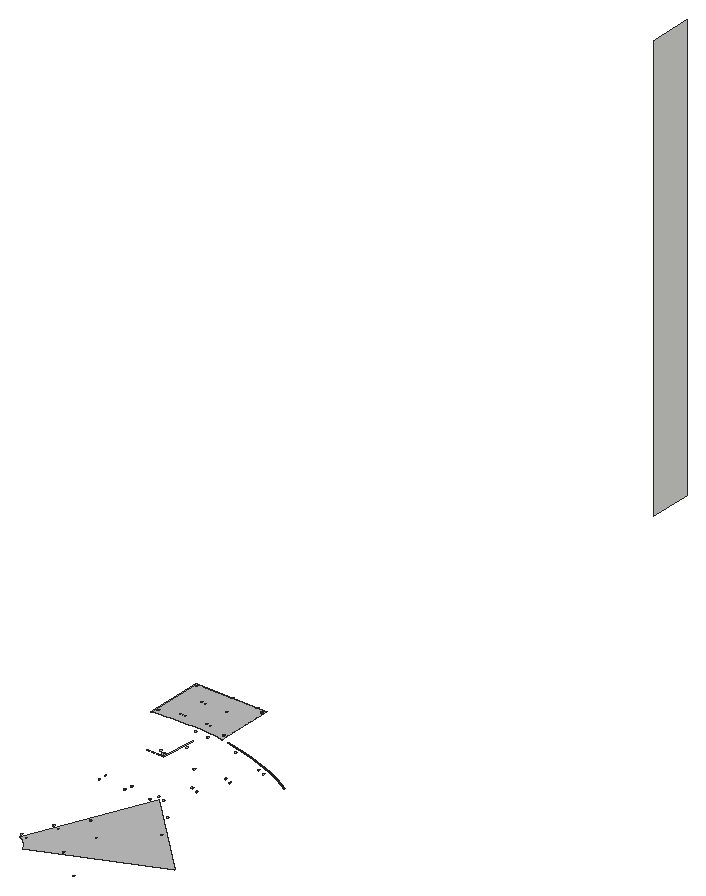
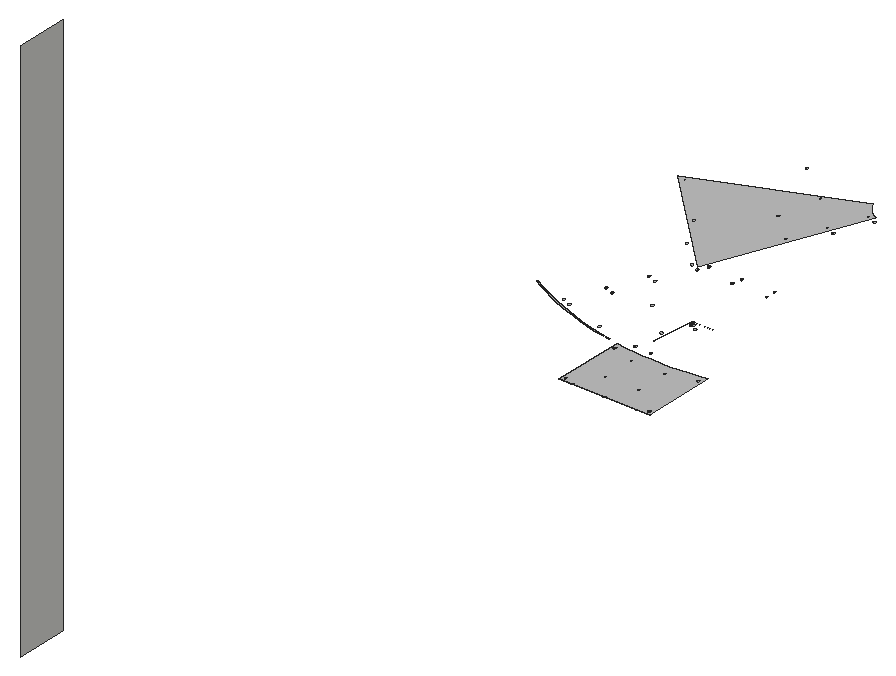
# SketchUp Ruby script. Lengths in inches.
U = 1.inch
M = Sketchup.active_model
def pt(a) = Geom::Point3d.new(a.map { |v| v * U })
def face(e, loops, mat)
  f = e.add_face(loops[0].map { |a| pt(a) })
  loops[1..].each { |l| e.add_face(l.map { |a| pt(a) }).erase! }
  f.material = f.back_material = mat if mat
  f
end
# faces: each face lists its corners as indices into pts; further lists are holes
def faces(e, pts, list, mat = nil) = list.each { |f| face(e, (f[0].is_a?(Array) ? f : [f]).map { |l| l.map { |i| pts[i] } }, mat) }
# xy, xz, yz: faces in a plane at the given z, y or x. An outline is a flat list of corners, or four numbers for a rectangle; further outlines are holes
def ring(l) = l.size == 4 ? [[l[0], l[1]], [l[2], l[1]], [l[2], l[3]], [l[0], l[3]]] : l.each_slice(2).to_a
def flat(e, list, mat, &to3) = list.each { |f| face(e, (f[0].is_a?(Array) ? f : [f]).map { |l| ring(l).map { |u, v| to3.(u, v) } }, mat) }
def xy(e, z, list, mat = nil) = flat(e, list, mat) { |x, y| [x, y, z] }
def xz(e, y, list, mat = nil) = flat(e, list, mat) { |x, z| [x, y, z] }
def yz(e, x, list, mat = nil) = flat(e, list, mat) { |y, z| [x, y, z] }
def lines(e, pts, list) = list.each { |a, b| e.add_line(pt(pts[a]), pt(pts[b])) }
# prism: a flat outline (further loops are holes) pulled along v
def prism(e, loops, v, mat = nil)
  f = face(e, loops, mat); d = Geom::Vector3d.new(v.map { |x| x * U })
  f.pushpull(f.normal.samedirection?(d) ? d.length : -d.length)
end
def box(e, o, s, mat = nil) = prism(e, [[o, [o[0] + s[0], o[1], o[2]], [o[0] + s[0], o[1] + s[1], o[2]], [o[0], o[1] + s[1], o[2]]]], [0, 0, s[2]], mat)
def at(x, y, z, deg = 0) = Geom::Transformation.translation(pt([x, y, z])) * Geom::Transformation.rotation(ORIGIN, Z_AXIS, deg.degrees)
def axes(o, x, y, z) = Geom::Transformation.new([*x, 0, *y, 0, *z, 0, *pt(o).to_a, 1])
def part(name) = M.definitions.add(name)
# library, detail: a bought-in or finely detailed component or shape, given as its bounding box
def library(name, o, s) = part(name).tap { |d| box(d.entities, o, s) }
def detail(e, o, s) = box(e.add_group.entities, o, s)
def put(e, d, t, mat = nil) = e.add_instance(d, t).tap { |i| i.material = mat if mat }
def group(e, t, mat = nil) = e.add_group.tap { |g| g.transformation = t; g.material = mat if mat }.entities
root = M.entities
M.materials.add("[Metal_Steel_Textured_White]").color = [191, 191, 191]
xy(root,3.625,[[158.645,163.377,158.648,163.4,158.657,163.422,158.671,163.44,158.689,163.454,158.711,163.463,158.734,163.466,158.757,163.463,158.778,163.454,158.797,163.44,158.811,163.422,158.82,163.4,158.823,163.377,158.822,163.377,158.819,163.4,158.81,163.421,158.796,163.44,158.778,163.454,158.757,163.462,158.734,163.465,158.711,163.462,158.69,163.454,158.672,163.44,158.658,163.421,158.649,163.4,158.646,163.377],[[152.277,164.396,152.205,164.555,152.123,164.708,152.031,164.856,151.929,164.998,151.819,165.132,151.7,165.259,151.573,165.378,151.438,165.489,151.297,165.59,151.149,165.682,150.995,165.764,150.836,165.836,156.019,178.348,164.789,169.578],[151.348,165.939,151.371,165.942,151.392,165.951,151.411,165.965,151.425,165.984,151.434,166.005,151.437,166.028,151.434,166.051,151.425,166.073,151.411,166.091,151.392,166.105,151.371,166.114,151.348,166.117,151.325,166.114,151.304,166.105,151.285,166.091,151.271,166.073,151.262,166.051,151.259,166.028,151.262,166.005,151.271,165.984,151.285,165.965,151.304,165.951,151.325,165.942],[156.159,177.554,156.182,177.557,156.204,177.566,156.222,177.58,156.236,177.599,156.245,177.62,156.248,177.643,156.245,177.666,156.236,177.688,156.222,177.706,156.204,177.72,156.182,177.729,156.159,177.732,156.136,177.729,156.115,177.72,156.096,177.706,156.082,177.688,156.073,177.666,156.07,177.643,156.073,177.62,156.082,177.599,156.096,177.58,156.115,177.566,156.136,177.557],[162.103,171.611,162.126,171.614,162.147,171.623,162.165,171.637,162.18,171.655,162.189,171.677,162.192,171.7,162.189,171.723,162.18,171.744,162.165,171.763,162.147,171.777,162.126,171.786,162.103,171.789,162.08,171.786,162.058,171.777,162.04,171.763,162.026,171.744,162.017,171.723,162.014,171.7,162.017,171.677,162.026,171.655,162.04,171.637,162.058,171.623,162.08,171.614],[154.956,174.651,154.979,174.654,155.001,174.663,155.019,174.677,155.033,174.695,155.042,174.717,155.045,174.74,155.042,174.763,155.033,174.784,155.019,174.802,155.001,174.817,154.979,174.825,154.956,174.828,154.933,174.825,154.912,174.817,154.893,174.802,154.879,174.784,154.87,174.763,154.867,174.74,154.87,174.717,154.879,174.695,154.893,174.677,154.912,174.663,154.933,174.654],[160.121,173.592,160.144,173.595,160.166,173.604,160.184,173.618,160.198,173.637,160.207,173.658,160.21,173.681,160.207,173.704,160.198,173.725,160.184,173.744,160.166,173.758,160.144,173.767,160.121,173.77,160.098,173.767,160.077,173.758,160.059,173.744,160.044,173.725,160.036,173.704,160.033,173.681,160.036,173.658,160.044,173.637,160.059,173.618,160.077,173.604,160.098,173.595],[153.754,171.747,153.777,171.75,153.798,171.759,153.816,171.773,153.831,171.791,153.839,171.813,153.842,171.836,153.839,171.859,153.831,171.88,153.816,171.899,153.798,171.913,153.777,171.922,153.754,171.925,153.731,171.922,153.709,171.913,153.691,171.899,153.677,171.88,153.668,171.859,153.665,171.836,153.668,171.813,153.677,171.791,153.691,171.773,153.709,171.759,153.731,171.75],[158.14,175.573,158.163,175.576,158.185,175.585,158.203,175.599,158.217,175.618,158.226,175.639,158.229,175.662,158.226,175.685,158.217,175.707,158.203,175.725,158.185,175.739,158.163,175.748,158.14,175.751,158.117,175.748,158.096,175.739,158.077,175.725,158.063,175.707,158.054,175.685,158.051,175.662,158.054,175.639,158.063,175.618,158.077,175.599,158.096,175.585,158.117,175.576],[155.372,166.021,155.395,166.024,155.417,166.033,155.435,166.047,155.449,166.066,155.458,166.087,155.461,166.11,155.458,166.133,155.449,166.155,155.435,166.173,155.417,166.187,155.395,166.196,155.372,166.199,155.349,166.196,155.328,166.187,155.31,166.173,155.295,166.155,155.287,166.133,155.284,166.11,155.287,166.087,155.295,166.066,155.31,166.047,155.328,166.033,155.349,166.024],[164.084,169.63,164.107,169.633,164.128,169.642,164.147,169.656,164.161,169.674,164.17,169.696,164.173,169.719,164.17,169.742,164.161,169.763,164.147,169.782,164.128,169.796,164.107,169.805,164.084,169.808,164.061,169.805,164.039,169.796,164.021,169.782,164.007,169.763,163.998,169.742,163.995,169.719,163.998,169.696,164.007,169.674,164.021,169.656,164.039,169.642,164.061,169.633],[152.469,164.819,152.492,164.822,152.513,164.831,152.532,164.845,152.546,164.863,152.555,164.885,152.558,164.908,152.555,164.931,152.546,164.952,152.532,164.97,152.513,164.984,152.492,164.993,152.469,164.996,152.446,164.993,152.424,164.984,152.406,164.97,152.392,164.952,152.383,164.931,152.38,164.908,152.383,164.885,152.392,164.863,152.406,164.845,152.424,164.831,152.446,164.822],[161.18,168.427,161.203,168.43,161.224,168.439,161.243,168.453,161.257,168.471,161.266,168.493,161.269,168.516,161.266,168.539,161.257,168.56,161.243,168.579,161.224,168.593,161.203,168.602,161.18,168.605,161.157,168.602,161.136,168.593,161.117,168.579,161.103,168.56,161.094,168.539,161.091,168.516,161.094,168.493,161.103,168.471,161.117,168.453,161.136,168.439,161.157,168.43],[152.551,168.843,152.574,168.846,152.595,168.855,152.614,168.869,152.628,168.888,152.637,168.909,152.64,168.932,152.637,168.955,152.628,168.976,152.614,168.995,152.595,169.009,152.574,169.018,152.551,169.021,152.528,169.018,152.506,169.009,152.488,168.995,152.474,168.976,152.465,168.955,152.462,168.932,152.465,168.909,152.474,168.888,152.488,168.869,152.506,168.855,152.528,168.846],[158.276,167.224,158.299,167.227,158.321,167.236,158.339,167.25,158.353,167.269,158.362,167.29,158.365,167.313,158.362,167.336,158.353,167.358,158.339,167.376,158.321,167.39,158.299,167.399,158.276,167.402,158.253,167.399,158.232,167.39,158.213,167.376,158.199,167.358,158.19,167.336,158.1875,167.313,158.19,167.29,158.199,167.269,158.213,167.25,158.232,167.236,158.253,167.227],[156.122,169.593,156.145,169.596,156.167,169.605,156.185,169.619,156.199,169.637,156.208,169.659,156.211,169.682,156.208,169.705,156.199,169.726,156.185,169.745,156.167,169.759,156.145,169.768,156.122,169.771,156.099,169.768,156.078,169.759,156.06,169.745,156.045,169.726,156.037,169.705,156.033,169.682,156.037,169.659,156.045,169.637,156.06,169.619,156.078,169.605,156.099,169.596]],[[151.348,165.992,151.339,165.993,151.33,165.996,151.322,166.002,151.316,166.01,151.3125,166.019,151.311,166.028,151.3125,166.038,151.316,166.046,151.322,166.054,151.33,166.06,151.339,166.064,151.348,166.065,151.357,166.064,151.366,166.06,151.374,166.054,151.38,166.046,151.383,166.038,151.385,166.028,151.383,166.019,151.38,166.01,151.374,166.002,151.366,165.996,151.357,165.993],[151.348,166.008,151.353,166.009,151.358,166.011,151.362,166.014,151.365,166.018,151.367,166.023,151.368,166.028,151.367,166.033,151.365,166.038,151.362,166.042,151.358,166.045,151.353,166.047,151.348,166.048,151.343,166.047,151.338,166.045,151.334,166.042,151.331,166.038,151.329,166.033,151.328,166.028,151.329,166.023,151.331,166.018,151.334,166.014,151.338,166.011,151.343,166.009]],[151.348,166.008,151.343,166.009,151.338,166.011,151.334,166.014,151.331,166.018,151.329,166.023,151.328,166.028,151.329,166.033,151.331,166.038,151.334,166.042,151.338,166.045,151.343,166.047,151.348,166.048,151.353,166.047,151.358,166.045,151.362,166.042,151.365,166.038,151.367,166.033,151.368,166.028,151.367,166.023,151.365,166.018,151.362,166.014,151.358,166.011,151.353,166.009],[[155.372,166.021,155.349,166.024,155.328,166.033,155.31,166.047,155.295,166.066,155.287,166.087,155.284,166.11,155.287,166.133,155.295,166.155,155.31,166.173,155.328,166.187,155.349,166.196,155.372,166.199,155.395,166.196,155.417,166.187,155.435,166.173,155.449,166.155,155.458,166.133,155.461,166.11,155.458,166.087,155.449,166.066,155.435,166.047,155.417,166.033,155.395,166.024],[155.372,166.022,155.395,166.025,155.416,166.034,155.435,166.048,155.449,166.066,155.457,166.088,155.46,166.11,155.457,166.133,155.449,166.154,155.435,166.172,155.416,166.186,155.395,166.195,155.372,166.198,155.35,166.195,155.328,166.186,155.31,166.172,155.296,166.154,155.288,166.133,155.285,166.11,155.288,166.088,155.296,166.066,155.31,166.048,155.328,166.034,155.35,166.025]],
  [[155.372,166.022,155.35,166.025,155.328,166.034,155.31,166.048,155.296,166.066,155.288,166.088,155.285,166.11,155.288,166.133,155.296,166.154,155.31,166.172,155.328,166.186,155.35,166.195,155.372,166.198,155.395,166.195,155.416,166.186,155.435,166.172,155.449,166.154,155.457,166.133,155.46,166.11,155.457,166.088,155.449,166.066,155.435,166.048,155.416,166.034,155.395,166.025],[155.372,166.074,155.382,166.075,155.391,166.079,155.398,166.084,155.404,166.092,155.408,166.101,155.409,166.11,155.408,166.12,155.404,166.129,155.398,166.136,155.391,166.142,155.382,166.146,155.372,166.147,155.363,166.146,155.354,166.142,155.347,166.136,155.341,166.129,155.337,166.12,155.336,166.11,155.337,166.101,155.341,166.092,155.347,166.084,155.354,166.079,155.363,166.075]],[[155.372,166.074,155.363,166.075,155.354,166.079,155.347,166.084,155.341,166.092,155.337,166.101,155.336,166.11,155.337,166.12,155.341,166.129,155.347,166.136,155.354,166.142,155.363,166.146,155.372,166.147,155.382,166.146,155.391,166.142,155.398,166.136,155.404,166.129,155.408,166.12,155.409,166.11,155.408,166.101,155.404,166.092,155.398,166.084,155.391,166.079,155.382,166.075],[155.372,166.09,155.378,166.091,155.382,166.093,155.387,166.096,155.39,166.1,155.392,166.105,155.392,166.115,155.39,166.12,155.387,166.124,155.382,166.128,155.378,166.13,155.367,166.13,155.362,166.128,155.358,166.124,155.355,166.12,155.353,166.115,155.352,166.11,155.353,166.105,155.355,166.1,155.358,166.096,155.362,166.093,155.367,166.091]],[155.372,166.09,155.367,166.091,155.362,166.093,155.358,166.096,155.355,166.1,155.353,166.105,155.352,166.11,155.353,166.115,155.355,166.12,155.358,166.124,155.362,166.128,155.367,166.13,155.378,166.13,155.382,166.128,155.387,166.124,155.39,166.12,155.392,166.115,155.392,166.105,155.39,166.1,155.387,166.096,155.382,166.093,155.378,166.091],[[150.61,166.245,150.587,166.248,150.566,166.257,150.547,166.271,150.533,166.289,150.524,166.311,150.521,166.334,150.524,166.357,150.533,166.378,150.547,166.397,150.566,166.411,150.587,166.42,150.61,166.423,150.633,166.42,150.655,166.411,150.673,166.397,150.6875,166.378,150.696,166.357,150.699,166.334,150.696,166.311,150.6875,166.289,150.673,166.271,150.655,166.257,150.633,166.248],[150.61,166.246,150.633,166.249,150.654,166.258,150.672,166.272,150.686,166.29,150.695,166.311,150.698,166.334,150.695,166.356,150.686,166.378,150.672,166.396,150.654,166.41,150.633,166.419,150.61,166.422,150.588,166.419,150.566,166.41,150.548,166.396,150.534,166.378,150.525,166.356,150.522,166.334,150.525,166.311,150.534,166.29,150.548,166.272,150.566,166.258,150.588,166.249]],[[152.551,168.895,152.541,168.897,152.532,168.9,152.525,168.906,152.519,168.914,152.515,168.923,152.514,168.932,152.515,168.941,152.519,168.95,152.525,168.958,152.532,168.964,152.541,168.967,152.551,168.969,152.56,168.967,152.569,168.964,152.577,168.958,152.582,168.95,152.586,168.941,152.587,168.932,152.586,168.923,152.582,168.914,152.577,168.906,152.569,168.9,152.56,168.897],[152.551,168.912,152.556,168.913,152.561,168.915,152.565,168.918,152.568,168.922,152.57,168.927,152.571,168.932,152.57,168.937,152.568,168.942,152.565,168.946,152.561,168.949,152.556,168.951,152.551,168.952,152.546,168.951,152.541,168.949,152.537,168.946,152.533,168.942,152.531,168.937,152.531,168.927,152.533,168.922,152.537,168.918,152.541,168.915,152.546,168.913]],
  [152.551,168.912,152.546,168.913,152.541,168.915,152.537,168.918,152.533,168.922,152.531,168.927,152.531,168.937,152.533,168.942,152.537,168.946,152.541,168.949,152.546,168.951,152.551,168.952,152.556,168.951,152.561,168.949,152.565,168.946,152.568,168.942,152.57,168.937,152.571,168.932,152.57,168.927,152.568,168.922,152.565,168.918,152.561,168.915,152.556,168.913],[[151.813,169.149,151.79,169.152,151.769,169.161,151.75,169.175,151.736,169.193,151.727,169.215,151.724,169.238,151.727,169.261,151.736,169.282,151.75,169.3,151.769,169.315,151.79,169.323,151.813,169.326,151.836,169.323,151.858,169.315,151.876,169.3,151.89,169.282,151.899,169.261,151.902,169.238,151.899,169.215,151.89,169.193,151.876,169.175,151.858,169.161,151.836,169.152],[151.813,169.15,151.836,169.153,151.857,169.161,151.875,169.175,151.889,169.194,151.898,169.215,151.901,169.238,151.898,169.26,151.889,169.281,151.875,169.3,151.857,169.314,151.836,169.322,151.813,169.325,151.79,169.322,151.769,169.314,151.751,169.3,151.737,169.281,151.728,169.26,151.725,169.238,151.728,169.215,151.737,169.194,151.751,169.175,151.769,169.161,151.79,169.153]],[[151.813,169.201,151.804,169.202,151.795,169.206,151.787,169.212,151.781,169.219,151.778,169.228,151.777,169.238,151.778,169.247,151.781,169.256,151.787,169.263,151.795,169.269,151.804,169.273,151.813,169.274,151.823,169.273,151.831,169.269,151.839,169.263,151.845,169.256,151.848,169.247,151.85,169.238,151.848,169.228,151.845,169.219,151.839,169.212,151.831,169.206,151.823,169.202],[151.808,169.218,151.818,169.218,151.823,169.22,151.827,169.223,151.83,169.228,151.832,169.232,151.833,169.238,151.832,169.243,151.83,169.248,151.827,169.252,151.823,169.255,151.818,169.257,151.808,169.257,151.803,169.255,151.799,169.252,151.796,169.248,151.794,169.243,151.793,169.238,151.794,169.232,151.796,169.228,151.799,169.223,151.803,169.22]],[[156.122,169.593,156.099,169.596,156.078,169.605,156.06,169.619,156.045,169.637,156.037,169.659,156.033,169.682,156.037,169.705,156.045,169.726,156.06,169.745,156.078,169.759,156.099,169.768,156.122,169.771,156.145,169.768,156.167,169.759,156.185,169.745,156.199,169.726,156.208,169.705,156.211,169.682,156.208,169.659,156.199,169.637,156.185,169.619,156.167,169.605,156.145,169.596],[156.122,169.594,156.145,169.597,156.166,169.606,156.185,169.62,156.199,169.638,156.207,169.659,156.21,169.682,156.207,169.705,156.199,169.726,156.185,169.744,156.166,169.758,156.145,169.767,156.122,169.77,156.1,169.767,156.078,169.758,156.06,169.744,156.046,169.726,156.037,169.705,156.034,169.682,156.037,169.659,156.046,169.638,156.06,169.62,156.078,169.606,156.1,169.597]],[[153.754,171.747,153.731,171.75,153.709,171.759,153.691,171.773,153.677,171.791,153.668,171.813,153.665,171.836,153.668,171.859,153.677,171.88,153.691,171.899,153.709,171.913,153.731,171.922,153.754,171.925,153.777,171.922,153.798,171.913,153.816,171.899,153.831,171.88,153.839,171.859,153.842,171.836,153.839,171.813,153.831,171.791,153.816,171.773,153.798,171.759,153.777,171.75],[153.754,171.748,153.776,171.751,153.798,171.76,153.816,171.774,153.83,171.792,153.838,171.813,153.841,171.836,153.838,171.859,153.83,171.88,153.816,171.898,153.798,171.912,153.776,171.921,153.754,171.924,153.731,171.921,153.71,171.912,153.691,171.898,153.677,171.88,153.669,171.859,153.666,171.836,153.669,171.813,153.677,171.792,153.691,171.774,153.71,171.76,153.731,171.751]],
  [[153.754,171.799,153.744,171.8,153.735,171.804,153.728,171.81,153.722,171.817,153.718,171.826,153.717,171.836,153.718,171.845,153.722,171.854,153.728,171.862,153.735,171.867,153.744,171.871,153.754,171.872,153.763,171.871,153.772,171.867,153.779,171.862,153.785,171.854,153.789,171.845,153.79,171.836,153.789,171.826,153.785,171.817,153.779,171.81,153.772,171.804,153.763,171.8],[153.748,171.816,153.759,171.816,153.764,171.818,153.768,171.822,153.771,171.826,153.773,171.831,153.774,171.836,153.773,171.841,153.771,171.846,153.768,171.85,153.764,171.853,153.759,171.855,153.754,171.856,153.748,171.855,153.744,171.853,153.739,171.85,153.736,171.846,153.734,171.841,153.734,171.831,153.736,171.826,153.739,171.822,153.744,171.818]],[153.748,171.816,153.744,171.818,153.739,171.822,153.736,171.826,153.734,171.831,153.734,171.841,153.736,171.846,153.739,171.85,153.744,171.853,153.748,171.855,153.754,171.856,153.759,171.855,153.764,171.853,153.768,171.85,153.771,171.846,153.773,171.841,153.774,171.836,153.773,171.831,153.771,171.826,153.768,171.822,153.764,171.818,153.759,171.816],[[160.121,173.593,160.099,173.596,160.078,173.605,160.059,173.619,160.045,173.637,160.037,173.658,160.034,173.681,160.037,173.704,160.045,173.725,160.059,173.743,160.078,173.757,160.099,173.766,160.121,173.769,160.144,173.766,160.165,173.757,160.184,173.743,160.198,173.725,160.206,173.704,160.209,173.681,160.206,173.658,160.198,173.637,160.184,173.619,160.165,173.605,160.144,173.596],[160.121,173.644,160.131,173.646,160.14,173.649,160.147,173.655,160.153,173.663,160.157,173.672,160.158,173.681,160.157,173.69,160.153,173.699,160.147,173.707,160.14,173.713,160.131,173.716,160.121,173.718,160.112,173.716,160.103,173.713,160.096,173.707,160.09,173.699,160.086,173.69,160.085,173.681,160.086,173.672,160.09,173.663,160.096,173.655,160.103,173.649,160.112,173.646]],[[158.588,176.255,158.565,176.258,158.544,176.267,158.525,176.281,158.511,176.299,158.502,176.321,158.499,176.344,158.502,176.367,158.511,176.388,158.525,176.407,158.544,176.421,158.565,176.43,158.588,176.433,158.611,176.43,158.632,176.421,158.651,176.407,158.665,176.388,158.674,176.367,158.677,176.344,158.674,176.321,158.665,176.299,158.651,176.281,158.632,176.267,158.611,176.258],[158.588,176.256,158.611,176.259,158.632,176.268,158.65,176.282,158.664,176.3,158.673,176.321,158.676,176.344,158.673,176.366,158.664,176.388,158.65,176.406,158.632,176.42,158.611,176.429,158.588,176.432,158.565,176.429,158.544,176.42,158.526,176.406,158.512,176.388,158.503,176.366,158.5,176.344,158.503,176.321,158.512,176.3,158.526,176.282,158.544,176.268,158.565,176.259]],[149.818,177.86,149.818,177.861,149.841,177.864,149.862,177.873,149.88,177.887,149.894,177.905,149.903,177.926,149.906,177.949,149.903,177.972,149.894,177.993,149.88,178.011,149.862,178.025,149.841,178.034,149.818,178.037,149.818,178.038,149.841,178.035,149.862,178.026,149.881,178.012,149.895,177.993,149.904,177.972,149.907,177.949,149.904,177.926,149.895,177.904,149.881,177.886,149.862,177.872,149.841,177.863],
  [[152.62,177.86,152.597,177.863,152.575,177.872,152.557,177.886,152.543,177.904,152.534,177.926,152.531,177.949,152.534,177.972,152.543,177.993,152.557,178.012,152.575,178.026,152.597,178.035,152.62,178.038,152.643,178.035,152.664,178.026,152.683,178.012,152.697,177.993,152.706,177.972,152.709,177.949,152.706,177.926,152.697,177.904,152.683,177.886,152.664,177.872,152.643,177.863],[152.62,177.861,152.642,177.864,152.664,177.873,152.682,177.887,152.696,177.905,152.705,177.926,152.708,177.949,152.705,177.972,152.696,177.993,152.682,178.011,152.664,178.025,152.642,178.034,152.62,178.037,152.597,178.034,152.576,178.025,152.558,178.011,152.544,177.993,152.535,177.972,152.532,177.949,152.535,177.926,152.544,177.905,152.558,177.887,152.576,177.873,152.597,177.864]],[[155.421,177.86,155.398,177.863,155.377,177.872,155.359,177.886,155.345,177.904,155.336,177.926,155.333,177.949,155.336,177.972,155.345,177.993,155.359,178.012,155.377,178.026,155.398,178.035,155.421,178.038,155.444,178.035,155.466,178.026,155.484,178.012,155.498,177.993,155.507,177.972,155.51,177.949,155.507,177.926,155.498,177.904,155.484,177.886,155.466,177.872,155.444,177.863],[155.421,177.861,155.444,177.864,155.465,177.873,155.484,177.887,155.498,177.905,155.506,177.926,155.509,177.949,155.506,177.972,155.498,177.993,155.484,178.011,155.465,178.025,155.444,178.034,155.421,178.037,155.399,178.034,155.378,178.025,155.359,178.011,155.345,177.993,155.337,177.972,155.334,177.949,155.337,177.926,155.345,177.905,155.359,177.887,155.378,177.873,155.399,177.864]],[149.818,177.861,149.818,177.912,149.827,177.914,149.836,177.917,149.844,177.923,149.85,177.931,149.853,177.939,149.854,177.949,149.853,177.958,149.85,177.967,149.844,177.975,149.836,177.981,149.827,177.984,149.818,177.985,149.818,178.037,149.841,178.034,149.862,178.025,149.88,178.011,149.894,177.993,149.903,177.972,149.906,177.949,149.903,177.926,149.894,177.905,149.88,177.887,149.862,177.873,149.841,177.864],[149.818,177.912,149.818,177.929,149.823,177.93,149.828,177.932,149.832,177.935,149.835,177.939,149.837,177.944,149.838,177.949,149.837,177.954,149.835,177.959,149.832,177.963,149.828,177.966,149.823,177.968,149.818,177.969,149.818,177.985,149.827,177.984,149.836,177.981,149.844,177.975,149.85,177.967,149.853,177.958,149.854,177.949,149.853,177.939,149.85,177.931,149.844,177.923,149.836,177.917,149.827,177.914],[[152.62,177.912,152.61,177.914,152.601,177.917,152.594,177.923,152.588,177.931,152.584,177.939,152.583,177.949,152.584,177.958,152.588,177.967,152.594,177.975,152.601,177.981,152.61,177.984,152.62,177.985,152.629,177.984,152.638,177.981,152.646,177.975,152.651,177.967,152.655,177.958,152.656,177.949,152.655,177.939,152.651,177.931,152.646,177.923,152.638,177.917,152.629,177.914],[152.62,177.929,152.625,177.93,152.63,177.932,152.634,177.935,152.637,177.939,152.639,177.944,152.64,177.949,152.639,177.954,152.637,177.959,152.634,177.963,152.63,177.966,152.625,177.968,152.62,177.969,152.615,177.968,152.61,177.966,152.606,177.963,152.602,177.959,152.6,177.954,152.6,177.944,152.602,177.939,152.606,177.935,152.61,177.932,152.615,177.93]],
  [[155.421,177.912,155.412,177.914,155.403,177.917,155.396,177.923,155.39,177.931,155.386,177.939,155.385,177.949,155.386,177.958,155.39,177.967,155.396,177.975,155.403,177.981,155.412,177.984,155.421,177.985,155.431,177.984,155.44,177.981,155.447,177.975,155.453,177.967,155.457,177.958,155.458,177.949,155.457,177.939,155.453,177.931,155.447,177.923,155.44,177.917,155.431,177.914],[155.421,177.929,155.427,177.93,155.431,177.932,155.436,177.935,155.439,177.939,155.441,177.944,155.441,177.954,155.439,177.959,155.436,177.963,155.431,177.966,155.427,177.968,155.421,177.969,155.416,177.968,155.412,177.966,155.407,177.963,155.404,177.959,155.402,177.954,155.402,177.944,155.404,177.939,155.407,177.935,155.412,177.932,155.416,177.93]],[152.62,177.929,152.615,177.93,152.61,177.932,152.606,177.935,152.602,177.939,152.6,177.944,152.6,177.954,152.602,177.959,152.606,177.963,152.61,177.966,152.615,177.968,152.62,177.969,152.625,177.968,152.63,177.966,152.634,177.963,152.637,177.959,152.639,177.954,152.64,177.949,152.639,177.944,152.637,177.939,152.634,177.935,152.63,177.932,152.625,177.93],[155.421,177.929,155.416,177.93,155.412,177.932,155.407,177.935,155.404,177.939,155.402,177.944,155.402,177.954,155.404,177.959,155.407,177.963,155.412,177.966,155.416,177.968,155.421,177.969,155.427,177.968,155.431,177.966,155.436,177.963,155.439,177.959,155.441,177.954,155.441,177.944,155.439,177.939,155.436,177.935,155.431,177.932,155.427,177.93],[[156.49,178.353,156.467,178.356,156.445,178.365,156.427,178.379,156.413,178.397,156.404,178.419,156.401,178.442,156.404,178.465,156.413,178.486,156.427,178.505,156.445,178.519,156.467,178.528,156.49,178.531,156.513,178.528,156.534,178.519,156.553,178.505,156.567,178.486,156.576,178.465,156.579,178.442,156.576,178.419,156.567,178.397,156.553,178.379,156.534,178.365,156.513,178.356],[156.49,178.354,156.513,178.357,156.534,178.366,156.552,178.38,156.566,178.398,156.575,178.419,156.578,178.442,156.575,178.465,156.566,178.486,156.552,178.504,156.534,178.518,156.513,178.527,156.49,178.53,156.467,178.527,156.446,178.518,156.428,178.504,156.414,178.486,156.405,178.465,156.402,178.442,156.405,178.419,156.414,178.398,156.428,178.38,156.446,178.366,156.467,178.357]],[[156.49,178.354,156.467,178.357,156.446,178.366,156.428,178.38,156.414,178.398,156.405,178.419,156.402,178.442,156.405,178.465,156.414,178.486,156.428,178.504,156.446,178.518,156.467,178.527,156.49,178.53,156.513,178.527,156.534,178.518,156.552,178.504,156.566,178.486,156.575,178.465,156.578,178.442,156.575,178.419,156.566,178.398,156.552,178.38,156.534,178.366,156.513,178.357],[156.49,178.405,156.499,178.406,156.508,178.41,156.516,178.416,156.522,178.423,156.525,178.432,156.526,178.442,156.525,178.451,156.522,178.46,156.516,178.468,156.508,178.473,156.499,178.477,156.49,178.478,156.48,178.477,156.472,178.473,156.464,178.468,156.458,178.46,156.455,178.451,156.453,178.442,156.455,178.432,156.458,178.423,156.464,178.416,156.472,178.41,156.48,178.406]],
  [[152.785,178.658,152.762,178.661,152.741,178.67,152.722,178.684,152.708,178.703,152.699,178.724,152.696,178.747,152.699,178.77,152.708,178.792,152.722,178.81,152.741,178.824,152.762,178.833,152.785,178.836,152.808,178.833,152.829,178.824,152.848,178.81,152.862,178.792,152.871,178.77,152.874,178.747,152.871,178.724,152.862,178.703,152.848,178.684,152.829,178.67,152.808,178.661],[152.785,178.659,152.808,178.662,152.829,178.671,152.847,178.685,152.861,178.703,152.87,178.725,152.873,178.747,152.87,178.77,152.861,178.791,152.847,178.809,152.829,178.823,152.808,178.832,152.785,178.835,152.762,178.832,152.741,178.823,152.723,178.809,152.709,178.791,152.7,178.77,152.697,178.747,152.7,178.725,152.709,178.703,152.723,178.685,152.741,178.671,152.762,178.662]],[[155.752,178.658,155.729,178.661,155.708,178.67,155.689,178.684,155.675,178.703,155.666,178.724,155.663,178.747,155.666,178.77,155.675,178.792,155.689,178.81,155.708,178.824,155.729,178.833,155.752,178.836,155.775,178.833,155.797,178.824,155.815,178.81,155.829,178.792,155.838,178.77,155.841,178.747,155.838,178.724,155.829,178.703,155.815,178.684,155.797,178.67,155.775,178.661],[155.752,178.659,155.775,178.662,155.796,178.671,155.814,178.685,155.828,178.703,155.837,178.725,155.84,178.747,155.837,178.77,155.828,178.791,155.814,178.809,155.796,178.823,155.775,178.832,155.752,178.835,155.729,178.832,155.708,178.823,155.69,178.809,155.676,178.791,155.667,178.77,155.664,178.747,155.667,178.725,155.676,178.703,155.69,178.685,155.708,178.671,155.729,178.662]],[149.818,178.659,149.818,178.711,149.827,178.712,149.836,178.716,149.844,178.721,149.85,178.729,149.853,178.738,149.854,178.747,149.853,178.757,149.85,178.766,149.844,178.773,149.836,178.779,149.827,178.783,149.818,178.784,149.818,178.835,149.841,178.832,149.862,178.823,149.88,178.809,149.894,178.791,149.903,178.77,149.906,178.747,149.903,178.725,149.894,178.703,149.88,178.685,149.862,178.671,149.841,178.662],[[152.785,178.711,152.776,178.712,152.767,178.716,152.759,178.721,152.753,178.729,152.75,178.738,152.748,178.747,152.75,178.757,152.753,178.766,152.759,178.773,152.767,178.779,152.776,178.783,152.785,178.784,152.795,178.783,152.803,178.779,152.811,178.773,152.817,178.766,152.82,178.757,152.822,178.747,152.82,178.738,152.817,178.729,152.811,178.721,152.803,178.716,152.795,178.712],[152.785,178.727,152.79,178.728,152.795,178.73,152.799,178.733,152.802,178.737,152.804,178.742,152.805,178.747,152.804,178.752,152.802,178.757,152.799,178.761,152.795,178.765,152.79,178.767,152.78,178.767,152.775,178.765,152.771,178.761,152.768,178.757,152.766,178.752,152.765,178.747,152.766,178.742,152.768,178.737,152.771,178.733,152.775,178.73,152.78,178.728]],[149.818,178.727,149.818,178.767,149.823,178.767,149.828,178.765,149.832,178.761,149.835,178.757,149.837,178.752,149.838,178.747,149.837,178.742,149.835,178.737,149.832,178.733,149.828,178.73,149.823,178.728],
  [152.785,178.727,152.78,178.728,152.775,178.73,152.771,178.733,152.768,178.737,152.766,178.742,152.765,178.747,152.766,178.752,152.768,178.757,152.771,178.761,152.775,178.765,152.78,178.767,152.79,178.767,152.795,178.765,152.799,178.761,152.802,178.757,152.804,178.752,152.805,178.747,152.804,178.742,152.802,178.737,152.799,178.733,152.795,178.73,152.79,178.728],[[157.732,181.353,157.709,181.356,157.688,181.365,157.67,181.379,157.656,181.397,157.647,181.419,157.644,181.442,157.647,181.465,157.656,181.486,157.67,181.505,157.688,181.519,157.709,181.528,157.732,181.531,157.755,181.528,157.777,181.519,157.795,181.505,157.809,181.486,157.818,181.465,157.821,181.442,157.818,181.419,157.809,181.397,157.795,181.379,157.777,181.365,157.755,181.356],[157.732,181.354,157.755,181.357,157.776,181.366,157.795,181.38,157.809,181.398,157.817,181.419,157.82,181.442,157.817,181.464,157.809,181.486,157.795,181.504,157.776,181.518,157.755,181.527,157.732,181.53,157.71,181.527,157.689,181.518,157.67,181.504,157.656,181.486,157.648,181.464,157.645,181.442,157.648,181.419,157.656,181.398,157.67,181.38,157.689,181.366,157.71,181.357]],[[157.732,181.405,157.723,181.406,157.714,181.41,157.707,181.416,157.701,181.423,157.697,181.432,157.696,181.442,157.697,181.451,157.701,181.46,157.707,181.468,157.714,181.473,157.723,181.477,157.732,181.478,157.742,181.477,157.751,181.473,157.758,181.468,157.764,181.46,157.768,181.451,157.769,181.442,157.768,181.432,157.764,181.423,157.758,181.416,157.751,181.41,157.742,181.406],[157.727,181.422,157.738,181.422,157.742,181.424,157.747,181.428,157.75,181.432,157.752,181.437,157.752,181.447,157.75,181.452,157.747,181.456,157.742,181.459,157.738,181.461,157.732,181.462,157.727,181.461,157.723,181.459,157.718,181.456,157.715,181.452,157.713,181.447,157.713,181.437,157.715,181.432,157.718,181.428,157.723,181.424]],[157.727,181.422,157.723,181.424,157.718,181.428,157.715,181.432,157.713,181.437,157.713,181.447,157.715,181.452,157.718,181.456,157.723,181.459,157.727,181.461,157.732,181.462,157.738,181.461,157.742,181.459,157.747,181.456,157.75,181.452,157.752,181.447,157.752,181.437,157.75,181.432,157.747,181.428,157.742,181.424,157.738,181.422],[[156.995,181.658,156.972,181.661,156.95,181.67,156.932,181.684,156.918,181.703,156.909,181.724,156.906,181.747,156.909,181.77,156.918,181.792,156.932,181.81,156.95,181.824,156.972,181.833,156.995,181.836,157.018,181.833,157.039,181.824,157.058,181.81,157.072,181.792,157.081,181.77,157.084,181.747,157.081,181.724,157.072,181.703,157.058,181.684,157.039,181.67,157.018,181.661],[156.995,181.659,157.018,181.662,157.039,181.671,157.057,181.685,157.071,181.703,157.08,181.725,157.083,181.747,157.08,181.77,157.071,181.791,157.057,181.809,157.039,181.823,157.018,181.832,156.995,181.835,156.972,181.832,156.951,181.823,156.933,181.809,156.919,181.791,156.91,181.77,156.907,181.747,156.91,181.725,156.919,181.703,156.933,181.685,156.951,181.671,156.972,181.662]],
  [[155.076,184.314,155.053,184.317,155.032,184.326,155.014,184.34,154.999,184.358,154.991,184.38,154.988,184.403,154.991,184.426,154.999,184.447,155.014,184.466,155.032,184.48,155.053,184.489,155.076,184.492,155.099,184.489,155.121,184.48,155.139,184.466,155.153,184.447,155.162,184.426,155.165,184.403,155.162,184.38,155.153,184.358,155.139,184.34,155.121,184.326,155.099,184.317],[155.076,184.315,155.099,184.318,155.12,184.327,155.139,184.341,155.153,184.359,155.161,184.38,155.164,184.403,155.161,184.426,155.153,184.447,155.139,184.465,155.12,184.479,155.099,184.488,155.076,184.491,155.054,184.488,155.033,184.479,155.014,184.465,155,184.447,154.992,184.426,154.989,184.403,154.992,184.38,155,184.359,155.014,184.341,155.033,184.327,155.054,184.318]],[[158.975,184.353,158.952,184.356,158.931,184.365,158.912,184.379,158.898,184.397,158.889,184.419,158.886,184.442,158.889,184.465,158.898,184.486,158.912,184.505,158.931,184.519,158.952,184.528,158.975,184.531,158.998,184.528,159.02,184.519,159.038,184.505,159.052,184.486,159.061,184.465,159.064,184.442,159.061,184.419,159.052,184.397,159.038,184.379,159.02,184.365,158.998,184.356],[158.975,184.354,158.998,184.357,159.019,184.366,159.037,184.38,159.051,184.398,159.06,184.419,159.063,184.442,159.06,184.464,159.051,184.486,159.037,184.504,159.019,184.518,158.998,184.527,158.975,184.53,158.952,184.527,158.931,184.518,158.913,184.504,158.899,184.486,158.89,184.464,158.887,184.442,158.89,184.419,158.899,184.398,158.913,184.38,158.931,184.366,158.952,184.357]],[[158.975,184.405,158.966,184.406,158.957,184.41,158.949,184.416,158.943,184.423,158.94,184.432,158.939,184.442,158.94,184.451,158.943,184.46,158.949,184.468,158.957,184.473,158.966,184.477,158.975,184.478,158.985,184.477,158.993,184.473,159.001,184.468,159.007,184.46,159.01,184.451,159.012,184.442,159.01,184.432,159.007,184.423,159.001,184.416,158.993,184.41,158.985,184.406],[158.97,184.422,158.98,184.422,158.985,184.424,158.989,184.428,158.992,184.432,158.994,184.437,158.995,184.442,158.994,184.447,158.992,184.452,158.989,184.456,158.985,184.459,158.98,184.461,158.975,184.462,158.97,184.461,158.965,184.459,158.961,184.456,158.958,184.452,158.956,184.447,158.955,184.442,158.956,184.437,158.958,184.432,158.961,184.428,158.965,184.424]],[158.97,184.422,158.965,184.424,158.961,184.428,158.958,184.432,158.956,184.437,158.955,184.442,158.956,184.447,158.958,184.452,158.961,184.456,158.965,184.459,158.97,184.461,158.975,184.462,158.98,184.461,158.985,184.459,158.989,184.456,158.992,184.452,158.994,184.447,158.995,184.442,158.994,184.437,158.992,184.432,158.989,184.428,158.985,184.424,158.98,184.422],[149.818,184.503,149.818,184.516,151.654,184.516,151.969,188.115,151.981,188.101,151.666,184.503],
  [[158.237,184.658,158.214,184.661,158.193,184.67,158.175,184.684,158.16,184.703,158.152,184.724,158.149,184.747,158.152,184.77,158.16,184.792,158.175,184.81,158.193,184.824,158.214,184.833,158.237,184.836,158.26,184.833,158.282,184.824,158.3,184.81,158.314,184.792,158.323,184.77,158.326,184.747,158.323,184.724,158.314,184.703,158.3,184.684,158.282,184.67,158.26,184.661],[158.237,184.659,158.26,184.662,158.281,184.671,158.3,184.685,158.314,184.703,158.322,184.724,158.325,184.747,158.322,184.77,158.314,184.791,158.3,184.809,158.281,184.823,158.26,184.832,158.237,184.835,158.215,184.832,158.193,184.823,158.175,184.809,158.161,184.791,158.153,184.77,158.15,184.747,158.153,184.724,158.161,184.703,158.175,184.685,158.193,184.671,158.215,184.662]],[[151.361,184.669,151.318,184.675,151.278,184.691,151.244,184.718,151.217,184.752,151.201,184.792,151.195,184.835,151.201,184.878,151.217,184.919,151.244,184.953,151.278,184.979,151.318,184.996,151.361,185.002,151.404,184.996,151.444,184.979,151.479,184.953,151.505,184.919,151.522,184.878,151.528,184.835,151.522,184.792,151.505,184.752,151.479,184.718,151.444,184.691,151.404,184.675],[151.361,184.716,151.392,184.72,151.421,184.732,151.446,184.751,151.465,184.776,151.477,184.804,151.481,184.835,151.477,184.866,151.465,184.895,151.446,184.92,151.421,184.939,151.392,184.951,151.361,184.955,151.33,184.951,151.301,184.939,151.277,184.92,151.258,184.895,151.246,184.866,151.242,184.835,151.246,184.804,151.258,184.776,151.277,184.751,151.301,184.732,151.33,184.72]],[[158.237,184.711,158.228,184.712,158.219,184.716,158.212,184.721,158.206,184.729,158.202,184.738,158.201,184.747,158.202,184.757,158.206,184.766,158.212,184.773,158.219,184.779,158.228,184.783,158.237,184.784,158.247,184.783,158.256,184.779,158.263,184.773,158.269,184.766,158.273,184.757,158.274,184.747,158.273,184.738,158.269,184.729,158.263,184.721,158.256,184.716,158.247,184.712],[158.237,184.727,158.243,184.728,158.247,184.73,158.252,184.733,158.255,184.737,158.257,184.742,158.257,184.752,158.255,184.757,158.252,184.761,158.247,184.765,158.243,184.767,158.232,184.767,158.227,184.765,158.223,184.761,158.22,184.757,158.218,184.752,158.217,184.747,158.218,184.742,158.22,184.737,158.223,184.733,158.227,184.73,158.232,184.728]],[158.237,184.727,158.232,184.728,158.227,184.73,158.223,184.733,158.22,184.737,158.218,184.742,158.217,184.747,158.218,184.752,158.22,184.757,158.223,184.761,158.227,184.765,158.232,184.767,158.243,184.767,158.247,184.765,158.252,184.761,158.255,184.757,158.257,184.752,158.257,184.742,158.255,184.737,158.252,184.733,158.247,184.73,158.243,184.728],[[150.816,185.093,150.793,185.096,150.772,185.105,150.754,185.119,150.74,185.137,150.731,185.159,150.728,185.181,150.731,185.204,150.74,185.225,150.754,185.244,150.772,185.258,150.793,185.266,150.816,185.269,150.839,185.266,150.86,185.258,150.878,185.244,150.892,185.225,150.901,185.204,150.904,185.181,150.901,185.159,150.892,185.137,150.878,185.119,150.86,185.105,150.839,185.096],[150.816,185.145,150.825,185.146,150.834,185.15,150.842,185.156,150.848,185.163,150.851,185.172,150.853,185.181,150.851,185.191,150.848,185.2,150.842,185.207,150.834,185.213,150.825,185.217,150.816,185.218,150.806,185.217,150.798,185.213,150.79,185.207,150.784,185.2,150.781,185.191,150.779,185.181,150.781,185.172,150.784,185.163,150.79,185.156,150.798,185.15,150.806,185.146]],
  [163.192,186.542,162.512,186.921,161.822,187.28,161.122,187.619,160.412,187.9375,159.694,188.235,158.967,188.512,158.232,188.767,157.49,189.001,156.742,189.213,155.987,189.404,155.228,189.572,154.475,189.716,154.464,189.718,154.475,189.784,155.241,189.637,156.003,189.469,156.759,189.278,157.509,189.065,158.253,188.83,158.99,188.574,159.718,188.297,160.439,187.998,161.15,187.679,161.852,187.339,162.544,186.979,163.225,186.599],[[152.279,186.841,152.256,186.844,152.235,186.853,152.217,186.867,152.203,186.885,152.194,186.906,152.191,186.929,152.194,186.952,152.203,186.973,152.217,186.991,152.235,187.005,152.256,187.014,152.279,187.017,152.302,187.014,152.323,187.005,152.341,186.991,152.355,186.973,152.364,186.952,152.367,186.929,152.364,186.906,152.355,186.885,152.341,186.867,152.323,186.853,152.302,186.844],[152.279,186.892,152.289,186.894,152.297,186.897,152.305,186.903,152.311,186.911,152.314,186.92,152.316,186.929,152.314,186.939,152.311,186.947,152.305,186.955,152.297,186.961,152.289,186.964,152.279,186.966,152.27,186.964,152.261,186.961,152.253,186.955,152.247,186.947,152.244,186.939,152.243,186.929,152.244,186.92,152.247,186.911,152.253,186.903,152.261,186.897,152.27,186.894]],[[160.218,187.353,160.195,187.356,160.173,187.365,160.155,187.379,160.141,187.397,160.132,187.419,160.129,187.442,160.132,187.465,160.141,187.486,160.155,187.505,160.173,187.519,160.195,187.528,160.218,187.531,160.241,187.528,160.262,187.519,160.281,187.505,160.295,187.486,160.304,187.465,160.307,187.442,160.304,187.419,160.295,187.397,160.281,187.379,160.262,187.365,160.241,187.356],[160.218,187.354,160.24,187.357,160.262,187.366,160.28,187.379,160.294,187.398,160.303,187.419,160.306,187.442,160.303,187.464,160.294,187.486,160.28,187.504,160.262,187.518,160.24,187.527,160.218,187.53,160.195,187.527,160.174,187.518,160.156,187.504,160.142,187.486,160.133,187.464,160.13,187.442,160.133,187.419,160.142,187.398,160.156,187.379,160.174,187.366,160.195,187.357]],[[159.48,187.659,159.457,187.662,159.436,187.671,159.418,187.685,159.404,187.703,159.395,187.724,159.392,187.747,159.395,187.77,159.404,187.791,159.418,187.809,159.436,187.823,159.457,187.832,159.48,187.835,159.503,187.832,159.524,187.823,159.542,187.809,159.556,187.791,159.565,187.77,159.568,187.747,159.565,187.724,159.556,187.703,159.542,187.685,159.524,187.671,159.503,187.662],[159.48,187.711,159.49,187.712,159.498,187.716,159.506,187.721,159.512,187.729,159.515,187.738,159.517,187.747,159.515,187.757,159.512,187.765,159.506,187.773,159.498,187.779,159.49,187.783,159.48,187.784,159.471,187.783,159.462,187.779,159.454,187.773,159.448,187.765,159.445,187.757,159.443,187.747,159.445,187.738,159.448,187.729,159.454,187.721,159.462,187.716,159.471,187.712]],[[156.049,188.753,156.026,188.756,156.004,188.764,155.986,188.779,155.972,188.797,155.963,188.818,155.96,188.841,155.963,188.864,155.972,188.886,155.986,188.904,156.004,188.918,156.026,188.927,156.049,188.93,156.072,188.927,156.093,188.918,156.112,188.904,156.126,188.886,156.135,188.864,156.138,188.841,156.135,188.818,156.126,188.797,156.112,188.779,156.093,188.764,156.072,188.756],[156.049,188.754,156.072,188.757,156.093,188.765,156.111,188.779,156.125,188.798,156.134,188.819,156.137,188.841,156.134,188.864,156.125,188.885,156.111,188.904,156.093,188.918,156.072,188.926,156.049,188.929,156.026,188.926,156.005,188.918,155.987,188.904,155.973,188.885,155.964,188.864,155.961,188.841,155.964,188.819,155.973,188.798,155.987,188.779,156.005,188.765,156.026,188.757]],
  [[152.5,189.366,152.477,189.369,152.456,189.378,152.437,189.392,152.423,189.411,152.414,189.432,152.411,189.455,152.414,189.478,152.423,189.5,152.437,189.518,152.456,189.532,152.477,189.541,152.5,189.544,152.523,189.541,152.545,189.532,152.563,189.518,152.577,189.5,152.586,189.478,152.589,189.455,152.586,189.432,152.577,189.411,152.563,189.392,152.545,189.378,152.523,189.369],[152.5,189.367,152.523,189.37,152.544,189.379,152.5625,189.393,152.576,189.411,152.585,189.432,152.588,189.455,152.585,189.478,152.576,189.499,152.5625,189.517,152.544,189.531,152.523,189.54,152.5,189.543,152.477,189.54,152.456,189.531,152.438,189.517,152.424,189.499,152.415,189.478,152.412,189.455,152.415,189.432,152.424,189.411,152.438,189.393,152.456,189.379,152.477,189.37]],[[152.5,189.419,152.491,189.42,152.482,189.423,152.474,189.429,152.468,189.437,152.465,189.446,152.464,189.455,152.465,189.465,152.468,189.473,152.474,189.481,152.482,189.487,152.491,189.491,152.5,189.492,152.51,189.491,152.518,189.487,152.526,189.481,152.532,189.473,152.535,189.465,152.537,189.455,152.535,189.446,152.532,189.437,152.526,189.429,152.518,189.423,152.51,189.42],[152.5,189.435,152.505,189.436,152.51,189.438,152.514,189.441,152.517,189.445,152.519,189.45,152.52,189.455,152.519,189.46,152.517,189.465,152.514,189.469,152.51,189.472,152.505,189.474,152.5,189.475,152.495,189.474,152.49,189.472,152.486,189.469,152.483,189.465,152.481,189.46,152.48,189.455,152.481,189.45,152.483,189.445,152.486,189.441,152.49,189.438,152.495,189.436]],[152.5,189.435,152.495,189.436,152.49,189.438,152.486,189.441,152.483,189.445,152.481,189.45,152.48,189.455,152.481,189.46,152.483,189.465,152.486,189.469,152.49,189.472,152.495,189.474,152.5,189.475,152.505,189.474,152.51,189.472,152.514,189.469,152.517,189.465,152.519,189.46,152.52,189.455,152.519,189.45,152.517,189.445,152.514,189.441,152.51,189.438,152.505,189.436],[[151.094,189.473,151.07,189.476,151.049,189.485,151.031,189.499,151.017,189.517,151.008,189.539,151.005,189.562,151.008,189.585,151.017,189.606,151.031,189.625,151.049,189.639,151.07,189.648,151.094,189.651,151.117,189.648,151.138,189.639,151.156,189.625,151.17,189.606,151.179,189.585,151.182,189.562,151.179,189.539,151.17,189.517,151.156,189.499,151.138,189.485,151.117,189.476],[151.094,189.474,151.116,189.477,151.137,189.486,151.156,189.5,151.17,189.518,151.178,189.539,151.181,189.562,151.178,189.584,151.17,189.606,151.156,189.624,151.137,189.638,151.116,189.647,151.094,189.65,151.071,189.647,151.05,189.638,151.031,189.624,151.017,189.606,151.009,189.584,151.006,189.562,151.009,189.539,151.017,189.518,151.031,189.5,151.05,189.486,151.071,189.477]],[[151.094,189.474,151.071,189.477,151.05,189.486,151.031,189.5,151.017,189.518,151.009,189.539,151.006,189.562,151.009,189.584,151.017,189.606,151.031,189.624,151.05,189.638,151.071,189.647,151.094,189.65,151.116,189.647,151.137,189.638,151.156,189.624,151.17,189.606,151.178,189.584,151.181,189.562,151.178,189.539,151.17,189.518,151.156,189.5,151.137,189.486,151.116,189.477],[151.094,189.525,151.103,189.526,151.112,189.53,151.119,189.536,151.125,189.543,151.129,189.552,151.13,189.562,151.129,189.571,151.125,189.58,151.119,189.588,151.112,189.593,151.103,189.597,151.094,189.598,151.084,189.597,151.075,189.593,151.068,189.588,151.062,189.58,151.058,189.571,151.057,189.562,151.058,189.552,151.062,189.543,151.068,189.536,151.075,189.53,151.084,189.526]],
  [145.933,189.907,145.933,196.108,147.043,196.108,147.043,196.074,145.967,196.074,145.967,189.911],[153.702,189.907,153.669,189.911,153.669,196.074,152.593,196.074,152.593,196.108,153.702,196.108],[[145.967,189.911,145.967,196.074,153.669,196.074,153.669,189.911,152.931,190.007,152.155,190.085,151.377,190.141,150.598,190.174,149.818,190.185,149.038,190.174,148.259,190.141,147.48,190.085,146.704,190.007],[146.244,190.425,146.27,190.429,146.294,190.439,146.315,190.454,146.331,190.475,146.341,190.499,146.344,190.525,146.341,190.551,146.331,190.575,146.315,190.596,146.294,190.612,146.27,190.622,146.244,190.625,146.218,190.622,146.194,190.612,146.173,190.596,146.158,190.575,146.148,190.551,146.144,190.525,146.148,190.499,146.158,190.475,146.173,190.454,146.194,190.439,146.218,190.429],[146.244,195.697,146.27,195.7,146.294,195.71,146.315,195.726,146.331,195.747,146.341,195.771,146.344,195.797,146.341,195.823,146.331,195.847,146.315,195.868,146.294,195.883,146.27,195.893,146.244,195.897,146.218,195.893,146.194,195.883,146.173,195.868,146.158,195.847,146.148,195.823,146.144,195.797,146.148,195.771,146.158,195.747,146.173,195.726,146.194,195.71,146.218,195.7],[153.392,190.425,153.418,190.429,153.442,190.439,153.462,190.454,153.478,190.475,153.488,190.499,153.492,190.525,153.488,190.551,153.478,190.575,153.462,190.596,153.442,190.612,153.418,190.622,153.392,190.625,153.366,190.622,153.342,190.612,153.321,190.596,153.305,190.575,153.295,190.551,153.292,190.525,153.295,190.499,153.305,190.475,153.321,190.454,153.342,190.439,153.366,190.429],[153.392,195.697,153.418,195.7,153.442,195.71,153.462,195.726,153.478,195.747,153.488,195.771,153.492,195.797,153.488,195.823,153.478,195.847,153.462,195.868,153.442,195.883,153.418,195.893,153.392,195.897,153.366,195.893,153.342,195.883,153.321,195.868,153.305,195.847,153.295,195.823,153.292,195.797,153.295,195.771,153.305,195.747,153.321,195.726,153.342,195.71,153.366,195.7],[150.928,193.91,151.483,193.966],[148.153,193.91,148.708,193.966],[150.928,191.135,151.483,191.191],[148.153,191.135,148.708,191.191]],[[146.244,190.425,146.218,190.429,146.194,190.439,146.173,190.454,146.158,190.475,146.148,190.499,146.144,190.525,146.148,190.551,146.158,190.575,146.173,190.596,146.194,190.612,146.218,190.622,146.244,190.625,146.27,190.622,146.294,190.612,146.315,190.596,146.331,190.575,146.341,190.551,146.344,190.525,146.341,190.499,146.331,190.475,146.315,190.454,146.294,190.439,146.27,190.429],[146.242,190.487,146.246,190.489,146.251,190.491,146.259,190.495,146.263,190.498,146.268,190.5,146.276,190.504,146.277,190.509,146.277,190.523,146.278,190.528,146.278,190.542,146.27,190.548,146.266,190.55,146.258,190.556,146.254,190.558,146.25,190.561,146.246,190.563,146.238,190.559,146.233,190.557,146.225,190.553,146.22,190.55,146.212,190.546,146.212,190.541,146.211,190.537,146.211,190.522,146.21,190.517,146.21,190.508,146.218,190.502,146.222,190.5,146.226,190.497,146.23,190.495,146.238,190.489]],[[153.392,190.425,153.366,190.429,153.342,190.439,153.321,190.454,153.305,190.475,153.295,190.499,153.292,190.525,153.295,190.551,153.305,190.575,153.321,190.596,153.342,190.612,153.366,190.622,153.392,190.625,153.418,190.622,153.442,190.612,153.462,190.596,153.478,190.575,153.488,190.551,153.492,190.525,153.488,190.499,153.478,190.475,153.462,190.454,153.442,190.439,153.418,190.429],[153.39,190.487,153.402,190.493,153.407,190.495,153.411,190.498,153.415,190.5,153.42,190.502,153.424,190.504,153.424,190.514,153.425,190.518,153.425,190.533,153.426,190.538,153.426,190.542,153.418,190.548,153.414,190.55,153.406,190.556,153.402,190.558,153.398,190.561,153.394,190.563,153.39,190.561,153.385,190.559,153.377,190.555,153.372,190.553,153.368,190.55,153.364,190.548,153.359,190.546,153.359,190.532,153.358,190.527,153.358,190.512,153.357,190.508,153.365,190.502,153.369,190.5,153.373,190.497,153.377,190.495,153.382,190.492,153.386,190.489]],
  [146.242,190.487,146.238,190.489,146.23,190.495,146.226,190.497,146.222,190.5,146.218,190.502,146.21,190.508,146.21,190.517,146.211,190.522,146.211,190.537,146.212,190.541,146.212,190.546,146.22,190.55,146.225,190.553,146.233,190.557,146.238,190.559,146.246,190.563,146.25,190.561,146.254,190.558,146.258,190.556,146.266,190.55,146.27,190.548,146.278,190.542,146.278,190.528,146.277,190.523,146.277,190.509,146.276,190.504,146.268,190.5,146.263,190.498,146.259,190.495,146.251,190.491,146.246,190.489],[153.39,190.487,153.386,190.489,153.382,190.492,153.377,190.495,153.373,190.497,153.369,190.5,153.365,190.502,153.357,190.508,153.358,190.512,153.358,190.527,153.359,190.532,153.359,190.546,153.364,190.548,153.368,190.55,153.372,190.553,153.377,190.555,153.385,190.559,153.39,190.561,153.394,190.563,153.398,190.561,153.402,190.558,153.406,190.556,153.414,190.55,153.418,190.548,153.426,190.542,153.426,190.538,153.425,190.533,153.425,190.518,153.424,190.514,153.424,190.504,153.42,190.502,153.415,190.5,153.411,190.498,153.407,190.495,153.402,190.493],[148.153,191.135,148.708,191.191],[150.928,191.135,151.483,191.191],[148.153,193.91,148.708,193.966],
  [150.928,193.91,151.483,193.966],[[146.244,195.697,146.218,195.7,146.194,195.71,146.173,195.726,146.158,195.747,146.148,195.771,146.144,195.797,146.148,195.823,146.158,195.847,146.173,195.868,146.194,195.883,146.218,195.893,146.244,195.897,146.27,195.893,146.294,195.883,146.315,195.868,146.331,195.847,146.341,195.823,146.344,195.797,146.341,195.771,146.331,195.747,146.315,195.726,146.294,195.71,146.27,195.7],[146.242,195.759,146.246,195.761,146.251,195.763,146.263,195.769,146.268,195.772,146.276,195.776,146.277,195.781,146.277,195.795,146.278,195.8,146.278,195.814,146.27,195.82,146.266,195.822,146.262,195.825,146.258,195.827,146.25,195.833,146.246,195.835,146.238,195.831,146.233,195.829,146.229,195.827,146.225,195.824,146.22,195.822,146.212,195.818,146.212,195.813,146.211,195.808,146.211,195.794,146.21,195.789,146.21,195.78,146.218,195.774,146.222,195.772,146.23,195.766,146.234,195.764,146.238,195.761]],[[153.392,195.697,153.366,195.7,153.342,195.71,153.321,195.726,153.305,195.747,153.295,195.771,153.292,195.797,153.295,195.823,153.305,195.847,153.321,195.868,153.342,195.883,153.366,195.893,153.392,195.897,153.418,195.893,153.442,195.883,153.462,195.868,153.478,195.847,153.488,195.823,153.492,195.797,153.488,195.771,153.478,195.747,153.462,195.726,153.442,195.71,153.418,195.7],[153.39,195.759,153.402,195.765,153.407,195.767,153.411,195.769,153.415,195.772,153.42,195.774,153.424,195.776,153.424,195.785,153.425,195.79,153.425,195.805,153.426,195.81,153.426,195.814,153.418,195.82,153.414,195.822,153.41,195.825,153.406,195.827,153.398,195.833,153.394,195.835,153.39,195.833,153.385,195.831,153.377,195.827,153.372,195.824,153.364,195.82,153.359,195.818,153.359,195.804,153.358,195.799,153.358,195.784,153.357,195.78,153.365,195.774,153.369,195.772,153.377,195.766,153.382,195.764,153.386,195.761]],[146.242,195.759,146.238,195.761,146.234,195.764,146.23,195.766,146.222,195.772,146.218,195.774,146.21,195.78,146.21,195.789,146.211,195.794,146.211,195.808,146.212,195.813,146.212,195.818,146.22,195.822,146.225,195.824,146.229,195.827,146.233,195.829,146.238,195.831,146.246,195.835,146.25,195.833,146.258,195.827,146.262,195.825,146.266,195.822,146.27,195.82,146.278,195.814,146.278,195.8,146.277,195.795,146.277,195.781,146.276,195.776,146.268,195.772,146.263,195.769,146.251,195.763,146.246,195.761],[153.39,195.759,153.386,195.761,153.382,195.764,153.377,195.766,153.369,195.772,153.365,195.774,153.357,195.78,153.358,195.784,153.358,195.799,153.359,195.804,153.359,195.818,153.364,195.82,153.372,195.824,153.377,195.827,153.385,195.831,153.39,195.833,153.394,195.835,153.398,195.833,153.406,195.827,153.41,195.825,153.414,195.822,153.418,195.82,153.426,195.814,153.426,195.81,153.425,195.805,153.425,195.79,153.424,195.785,153.424,195.776,153.42,195.774,153.415,195.772,153.411,195.769,153.407,195.767,153.402,195.765],
  [147.043,196.074,149.818,196.108],[149.818,196.074,152.593,196.108]],"[Metal_Steel_Textured_White]")
yz(root,158.149,[[243.402,3.625,247.965,50.25]])
